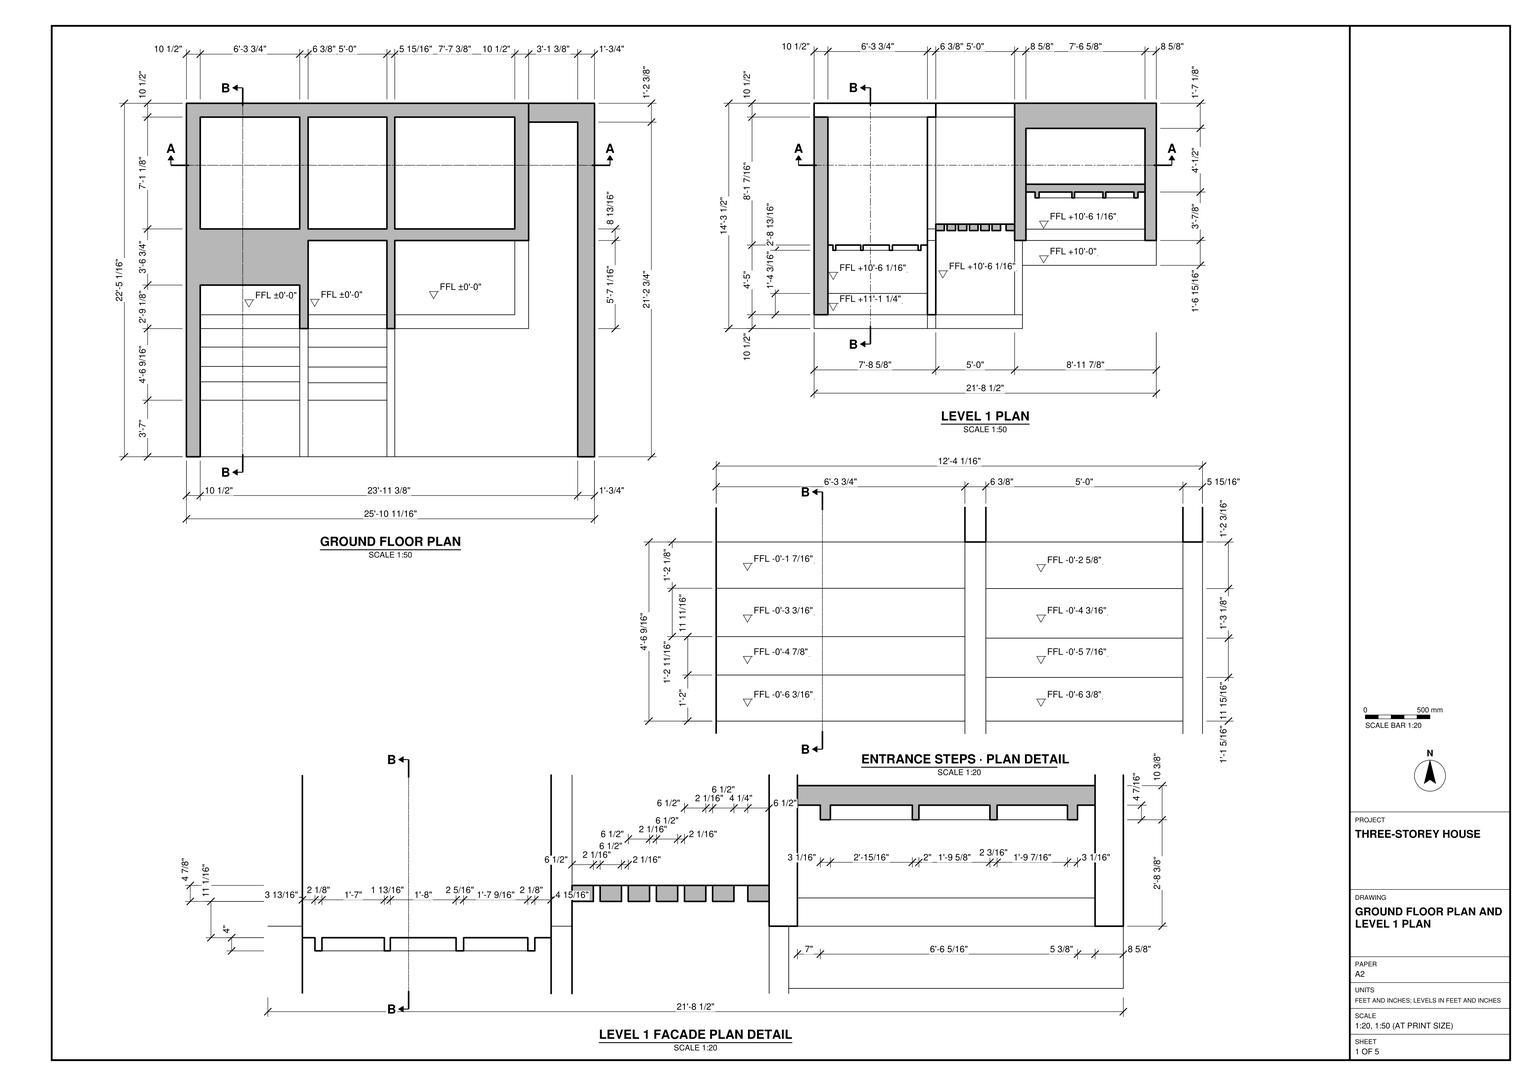
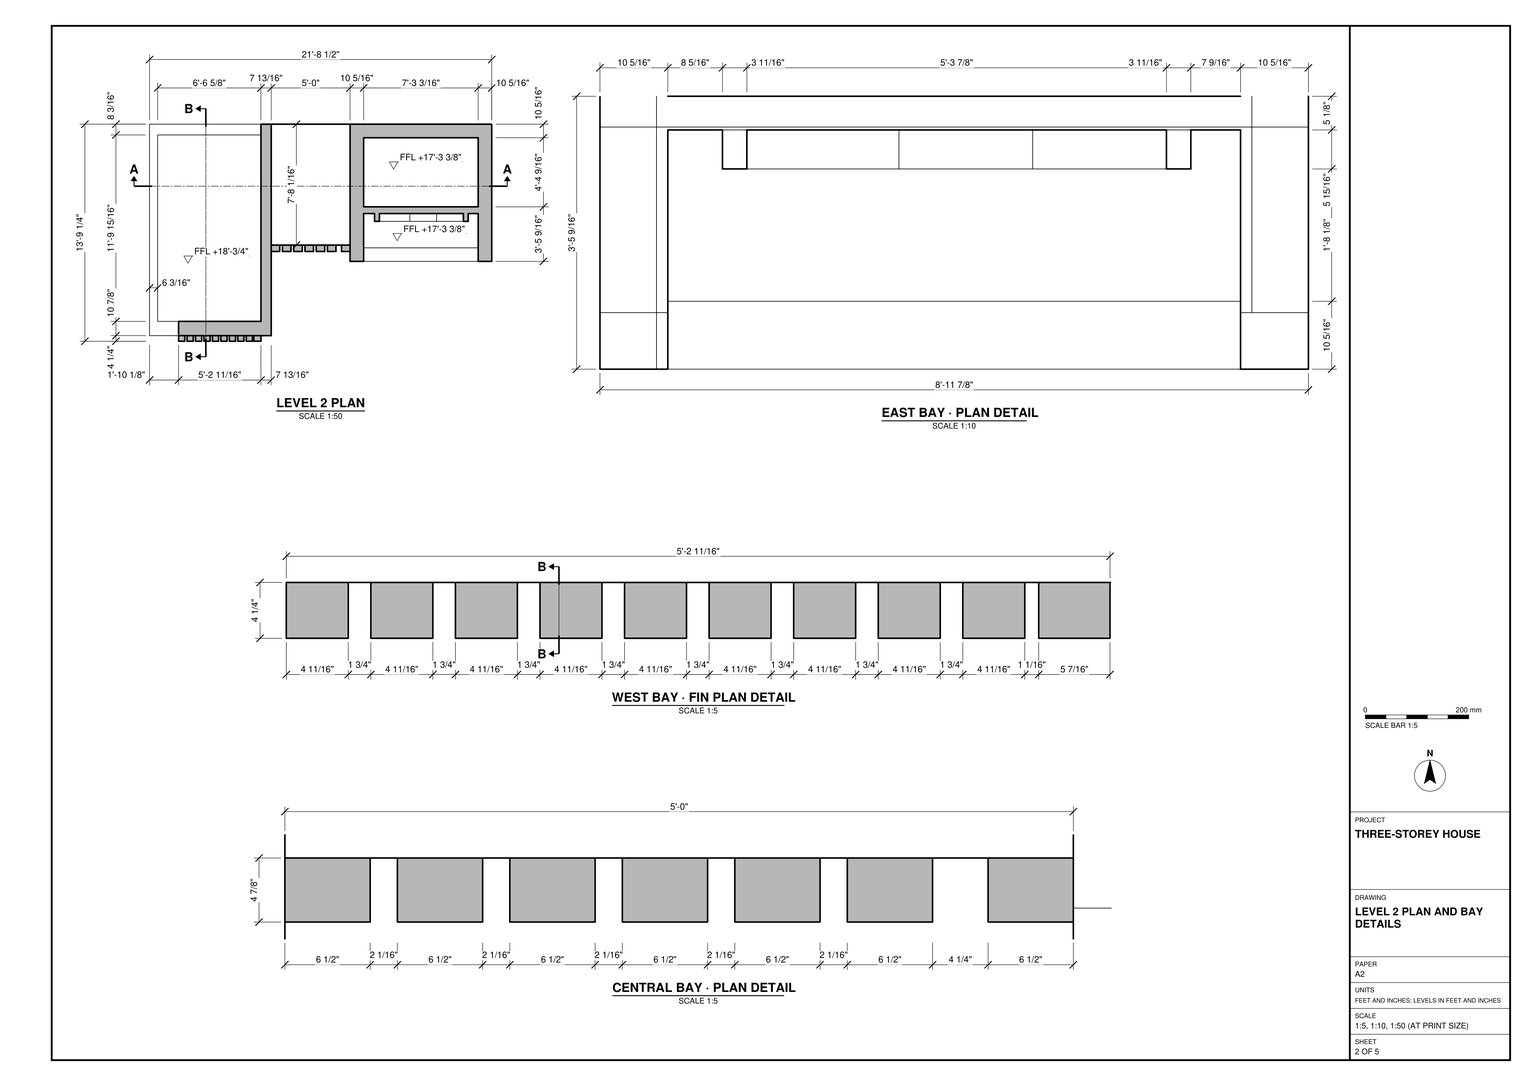
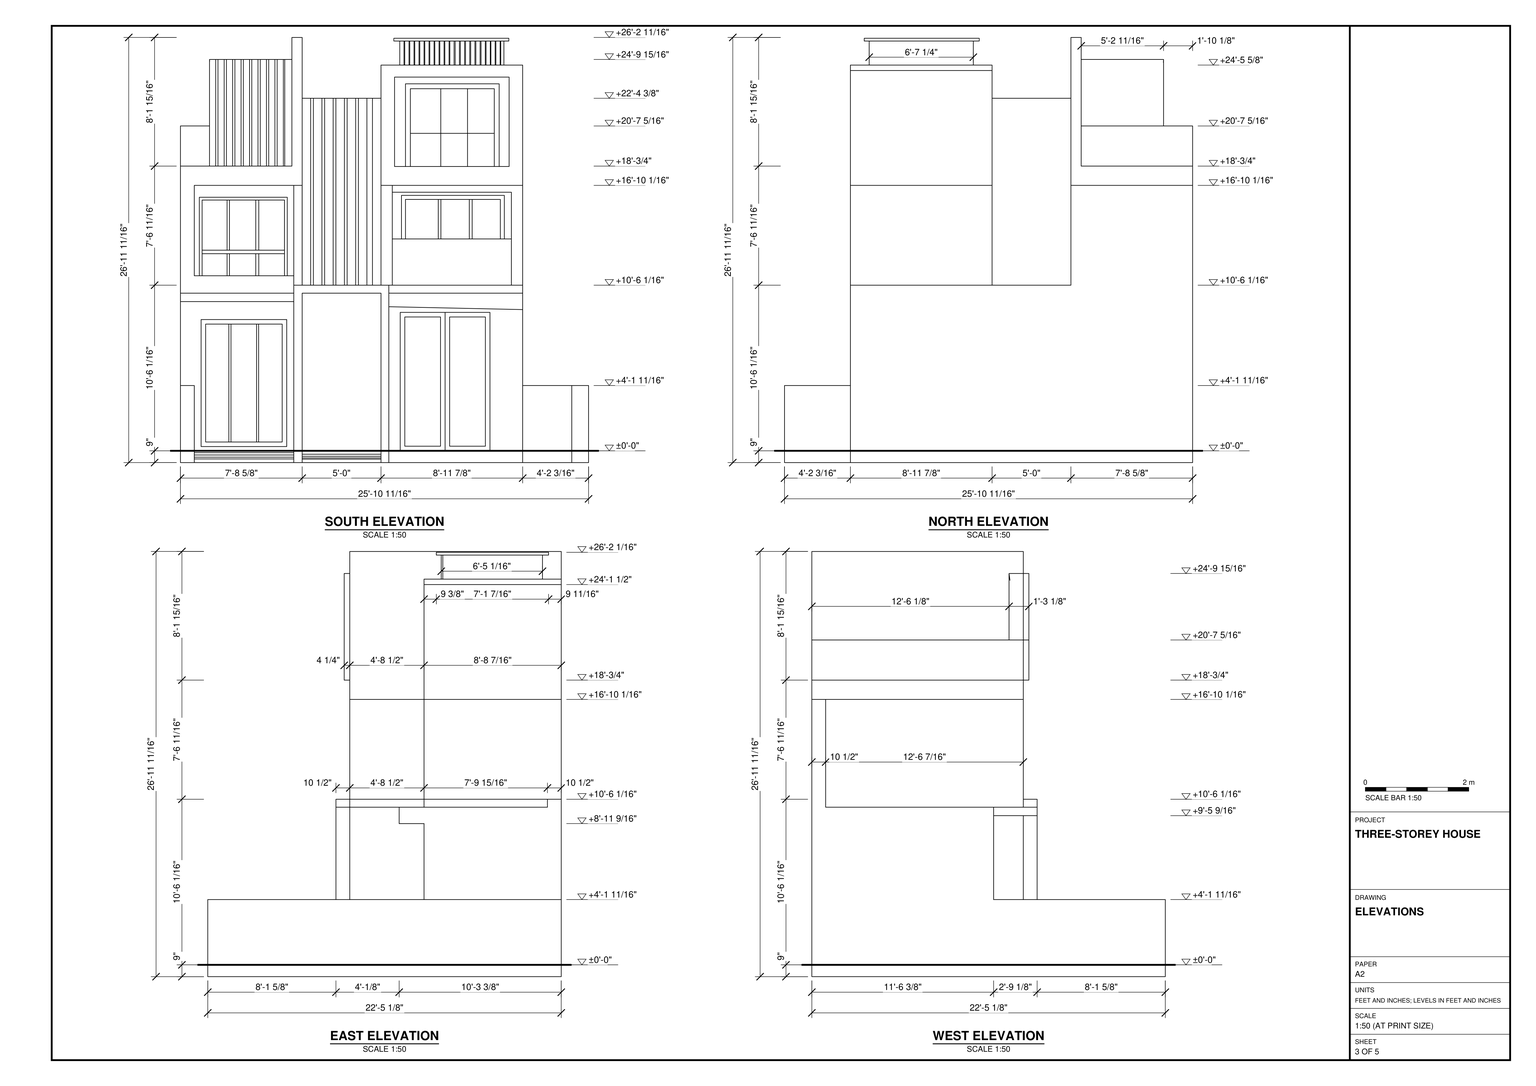
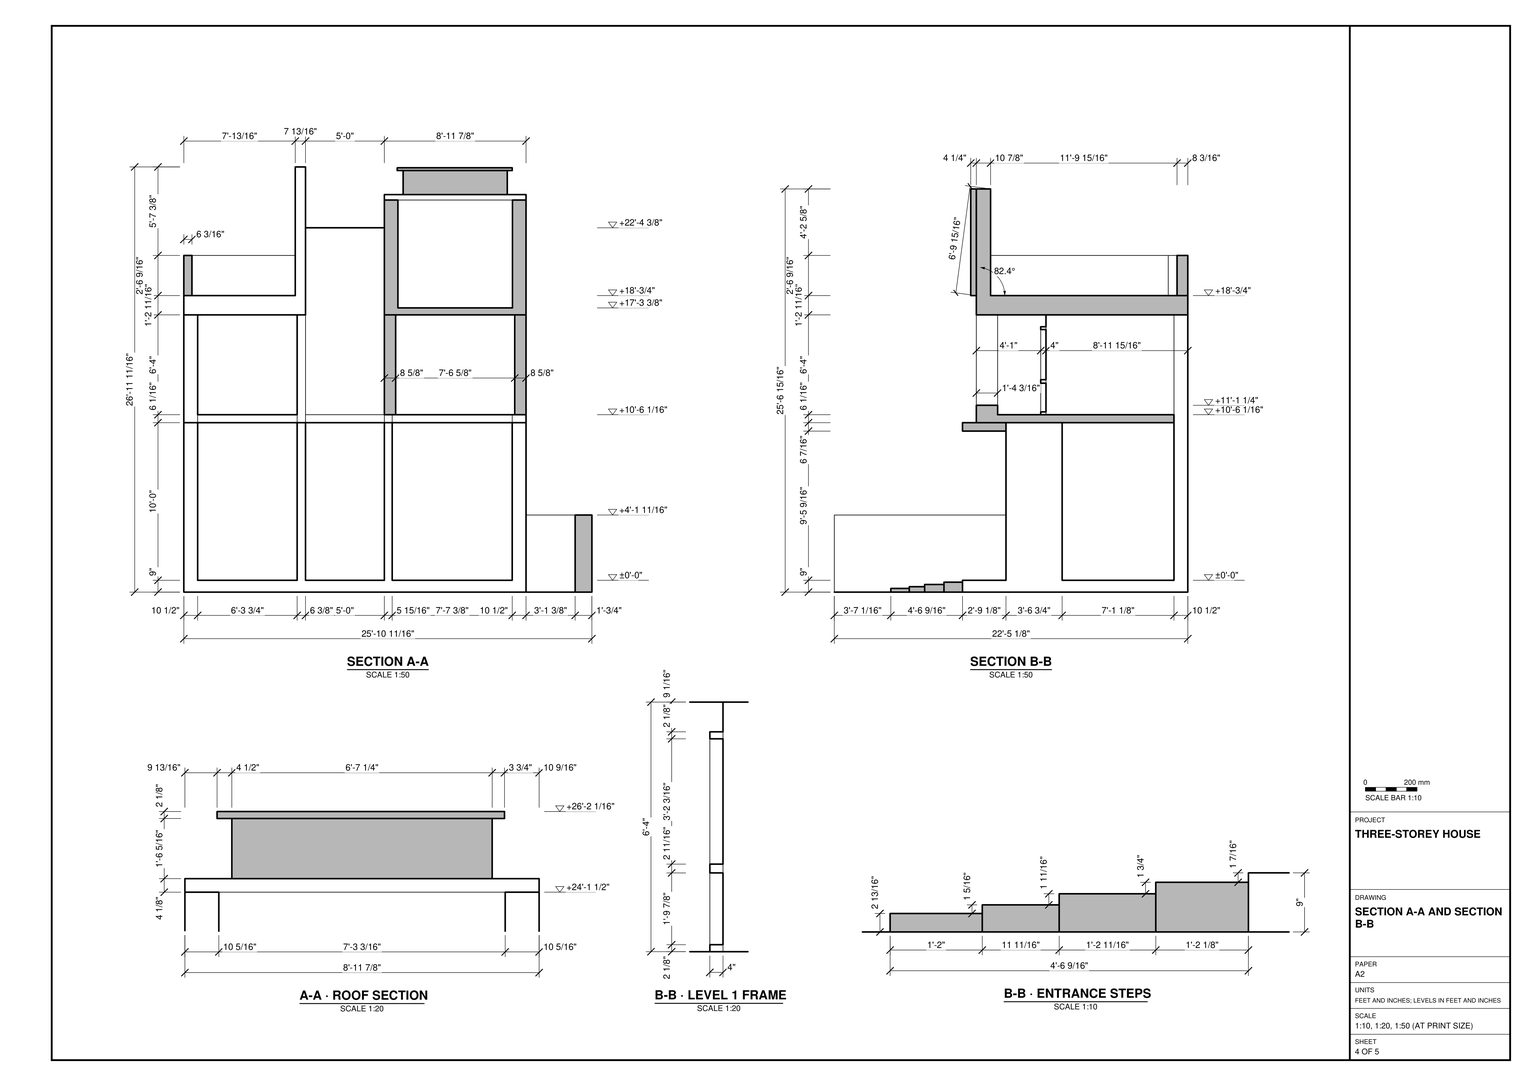
Build the three-storey house shown in task_files/diagram_01.pdf. Work in feet and inches. The overall width is 25'-10 11/16" east to west, the depth is 22'-5 1/16" north to south, and the height from the bottom of the base to the highest point is 26'-11 11/16". Set the ground floor at ±0'-0", Level 1 at +10'-6 1/16", and Level 2 at +18'-3/4".

Start with the ground-floor plan, including the base, the walls flanking the forecourt, and the two adjacent runs of shallow entrance steps. Use the wall thicknesses and partition positions drawn on each plan. Model the floor slabs and follow the stepped outline of the upper floors: the west bay projects furthest south, the centre bay is recessed from it, and the east bay sits further back. Use the south elevation for the arrangement of framed doors and windows, the solid panels below the upper glazing, and the vertical fins. Follow the bay details for the depth and spacing of the fins. Finish the roof with the different wall heights and the raised, capped detail over the east bay.

Keep walls, slabs, stairs, and roof elements in separate groups or components. Keep each furniture or joinery piece shown separate, and use components for repeated parts such as fins. Any decor or loose items shown may be represented by suitable library components. Save one SketchUp model as output_files/three_storey_house_with_stepped_bays_and_facade_fins.skp.

# SketchUp Ruby script. Lengths in inches.
U = 1.inch
M = Sketchup.active_model
def pt(a) = Geom::Point3d.new(a.map { |v| v * U })
def face(e, loops, mat)
  f = e.add_face(loops[0].map { |a| pt(a) })
  loops[1..].each { |l| e.add_face(l.map { |a| pt(a) }).erase! }
  f.material = f.back_material = mat if mat
  f
end
# faces: each face lists its corners as indices into pts; further lists are holes
def faces(e, pts, list, mat = nil) = list.each { |f| face(e, (f[0].is_a?(Array) ? f : [f]).map { |l| l.map { |i| pts[i] } }, mat) }
# xy, xz, yz: faces in a plane at the given z, y or x. An outline is a flat list of corners, or four numbers for a rectangle; further outlines are holes
def ring(l) = l.size == 4 ? [[l[0], l[1]], [l[2], l[1]], [l[2], l[3]], [l[0], l[3]]] : l.each_slice(2).to_a
def flat(e, list, mat, &to3) = list.each { |f| face(e, (f[0].is_a?(Array) ? f : [f]).map { |l| ring(l).map { |u, v| to3.(u, v) } }, mat) }
def xy(e, z, list, mat = nil) = flat(e, list, mat) { |x, y| [x, y, z] }
def xz(e, y, list, mat = nil) = flat(e, list, mat) { |x, z| [x, y, z] }
def yz(e, x, list, mat = nil) = flat(e, list, mat) { |y, z| [x, y, z] }
def lines(e, pts, list) = list.each { |a, b| e.add_line(pt(pts[a]), pt(pts[b])) }
# prism: a flat outline (further loops are holes) pulled along v
def prism(e, loops, v, mat = nil)
  f = face(e, loops, mat); d = Geom::Vector3d.new(v.map { |x| x * U })
  f.pushpull(f.normal.samedirection?(d) ? d.length : -d.length)
end
def box(e, o, s, mat = nil) = prism(e, [[o, [o[0] + s[0], o[1], o[2]], [o[0] + s[0], o[1] + s[1], o[2]], [o[0], o[1] + s[1], o[2]]]], [0, 0, s[2]], mat)
def at(x, y, z, deg = 0) = Geom::Transformation.translation(pt([x, y, z])) * Geom::Transformation.rotation(ORIGIN, Z_AXIS, deg.degrees)
def axes(o, x, y, z) = Geom::Transformation.new([*x, 0, *y, 0, *z, 0, *pt(o).to_a, 1])
def part(name) = M.definitions.add(name)
# library, detail: a bought-in or finely detailed component or shape, given as its bounding box
def library(name, o, s) = part(name).tap { |d| box(d.entities, o, s) }
def detail(e, o, s) = box(e.add_group.entities, o, s)
def put(e, d, t, mat = nil) = e.add_instance(d, t).tap { |i| i.material = mat if mat }
def group(e, t, mat = nil) = e.add_group.tap { |g| g.transformation = t; g.material = mat if mat }.entities
root = M.entities
M.materials.add("[Basic Tile]").color = [203, 206, 202]
M.materials.add("[Blinds Vertical Stripe Gray]").color = [160, 160, 160]
M.materials.add("[Color C01]").color = [255, 229, 204]
M.materials.add("[Formica Graystone]").color = [178, 174, 161]
M.materials.add("[Formica Graystone]1").color = [201, 197, 182]
M.materials.add("[Formica Graystone]3").color = [149, 146, 135]
M.materials.add("[Formica Laminate Dark]").color = [50, 53, 60]
M.materials.add("[Formica Speckled Grey]").color = [94, 105, 111]
M.materials.add("[Terrazzo Tile Light]").color = [219, 217, 210]
M.materials.add("[Translucent Glass Blue]").color = [100, 149, 237]
M.materials["[Translucent Glass Blue]"].alpha = 0.5
M.materials.add("[Translucent Glass Safety]").color = [204, 235, 244]
M.materials["[Translucent Glass Safety]"].alpha = 0.5
M.materials.add("[Translucent Glass Sky Reflection]").color = [126, 138, 183]
M.materials["[Translucent Glass Sky Reflection]"].alpha = 0.52
M.materials.add("[Vegetation Grass Artificial]").color = [98, 140, 74]
M.materials.add("[Wood Cherry Original]").color = [152, 86, 42]
M.materials.add("[Wood Veneer 01]").color = [79, 46, 24]
xy(root,0,[[0,0,0,269.09,260.51,269.09,260.51,97.58,10.52,97.58,10.52,0],[297.89,0,297.89,254.74,260.51,254.74,260.51,269.09,310.66,269.09,310.66,0],[10.52,43.03,86.27,57.06],[92.65,43.03,152.65,56.34],[92.65,56.34,152.65,68.3],
  [10.52,57.06,86.27,68.77],[92.65,68.3,152.65,83.4],[10.52,68.77,86.27,83.48],[92.65,83.4,152.65,97.58],[10.52,83.48,86.27,97.58]])
xy(root,0,[[10.52,0,86.27,43.03],[86.27,0,92.65,97.58],[92.65,0,152.65,43.03],[152.65,0,158.61,97.58],[158.61,0,158.61,97.58,260.51,97.58,260.51,254.74,297.89,254.74,297.89,0]],"[Vegetation Grass Artificial]")
xy(root,2.625,[[92.65,43.03,152.65,56.34]],"[Basic Tile]")
xy(root,2.8125,[[10.52,43.03,86.27,57.06]],"[Basic Tile]")
xy(root,3.5625,[[92.65,56.34,152.65,68.3]],"[Basic Tile]")
xy(root,4.125,[[10.52,57.06,86.27,68.77]],"[Basic Tile]")
xy(root,4.8125,[[92.65,68.3,152.65,83.4]],"[Basic Tile]")
xy(root,5.8125,[[10.52,68.77,86.27,83.48]],"[Basic Tile]")
xy(root,6.375,[[92.65,83.4,152.65,97.58]],"[Basic Tile]")
xy(root,7.5625,[[10.52,83.48,86.27,97.58]],"[Basic Tile]")
xy(root,9,[[10.52,173.43,86.27,258.57],[92.65,173.43,152.65,258.57],[158.61,173.43,249.99,258.57]])
xy(root,9,[[10.52,97.58,86.27,108.11],[92.65,97.58,152.65,108.11],[10.52,108.11,86.27,130.69]],"[Basic Tile]")
xy(root,9,[[92.65,108.11,152.65,164.63]],"[Color C01]")
xy(root,9,[[158.61,97.58,260.51,97.58,260.51,164.63,249.99,164.63,249.99,108.11,158.61,108.11],[158.61,108.11,249.99,164.63]],"[Terrazzo Tile Light]")
xy(root,58.6875,[[0,0,10.52,130.69],[297.89,0,310.66,0,310.66,269.09,260.51,269.09,260.51,254.74,297.89,254.74]],"[Terrazzo Tile Light]")
xy(root,122.58,[[0,97.58,86.27,130.69]])
xy(root,129,[[92.65,97.58,152.65,108.11],[0,108.11,86.27,130.69],[86.27,108.11,92.65,164.63],[92.65,108.11,152.65,164.63],[0,130.69,86.27,164.63],
  [0,164.63,260.51,173.43],[0,173.43,10.52,258.57],[10.52,173.43,86.27,258.57],[86.27,173.43,92.65,258.57],[92.65,173.43,152.65,258.57],
  [152.65,173.43,158.61,258.57],[158.61,173.43,249.99,258.57],[249.99,173.43,260.51,258.57]])
xy(root,129,[[0,97.58,86.27,108.11],[152.65,108.11,158.61,164.63],[158.61,145.69,260.51,164.63]],"[Color C01]")
xy(root,135.0625,[[14.35,157.13,81.31,157.13,81.31,161.13,86.27,161.13,86.27,258.57,10.52,258.57,10.52,161.13,14.35,161.13],[152.65,164.63,152.65,258.57,260.51,258.57,260.51,164.63,251.9,164.63,251.9,249.96,161.26,249.96,161.26,164.63],[161.26,164.63,251.9,173.24],[92.63,172.17,99.12,177.05],[101.19,172.17,107.68,177.05],
  [109.75,172.17,116.25,177.05],[118.32,172.17,124.81,177.05],[126.88,172.17,133.37,177.05],[135.44,172.17,141.93,177.05],[146.16,172.17,152.65,177.05],
  [161.26,173.24,251.9,201.49],[161.26,207.44,251.9,249.96],[92.65,258.57,152.65,269.09],[152.65,258.57,158.61,269.09],[158.61,258.57,249.99,269.09],
  [249.99,258.57,260.51,269.09]])
xy(root,135.0625,[[86.27,97.58,92.62,108.11],[92.62,97.58,158.61,108.11],[92.62,108.11,152.65,108.11,152.65,172.17,146.16,172.17,146.16,177.05,141.93,177.05,141.93,172.17,135.44,172.17,135.44,177.05,133.37,177.05,133.37,172.17,126.88,172.17,126.88,177.05,124.81,177.05,124.81,172.17,118.32,172.17,118.32,177.05,116.25,177.05,116.25,172.17,109.75,172.17,109.75,177.05,107.68,177.05,107.68,172.17,101.19,172.17,101.19,177.05,99.12,177.05,99.12,172.17,92.63,172.17],[10.52,124.32,86.27,124.32,86.27,161.13,81.31,161.13,81.31,157.13,14.35,157.13,14.35,161.13,10.52,161.13]],"[Color C01]")
xy(root,137.12,[[168.24,197.05,246.55,201.49]])
xy(root,137.19,[[16.48,157.13,35.48,161.13],[37.3,157.13,57.33,161.13],[59.62,157.13,79.18,161.13]],"[Wood Veneer 01]")
xy(root,140.17,[[171.3,197.05,196.26,201.49],[198.27,197.05,219.88,201.49],[222.0625,197.05,243.5,201.49]],"[Wood Veneer 01]")
xy(root,142.25,[[10.52,108.11,86.27,124.32]],"[Color C01]")
xy(root,159.05,[[16.48,157.13,35.48,161.13],[37.3,157.13,57.33,161.13],[59.62,157.13,79.18,161.13]])
xy(root,161.73,[[16.48,157.13,35.48,161.13],[37.3,157.13,57.33,161.13],[59.62,157.13,79.18,161.13]],"[Wood Veneer 01]")
xy(root,170.28,[[161.26,164.63,251.9,173.24]],"[Translucent Glass Safety]")
xy(root,199.89,[[16.48,157.13,35.48,161.13],[37.3,157.13,57.33,161.13],[59.62,157.13,79.18,161.13]],"[Wood Veneer 01]")
xy(root,200.375,[[171.3,197.05,196.26,201.49],[198.27,197.05,219.88,201.49],[222.0625,197.05,243.5,201.49]])
xy(root,202.01,[[14.35,157.13,81.31,161.13]],"[Wood Veneer 01]")
xy(root,203.43,[[168.24,197.05,246.55,201.49]],"[Wood Veneer 01]")
xy(root,205.84,[[161.26,164.63,251.9,173.24]],"[Wood Cherry Original]")
xy(root,211.0625,[[86.27,108.11,92.62,124.32],[92.62,108.11,92.63,124.32],[0,124.32,10.52,258.57],[86.27,124.32,92.62,124.32,92.63,172.17,92.63,258.57,86.27,258.57],[92.62,124.32,92.63,172.17,92.63,124.32],
  [10.52,161.13,86.27,161.13,86.27,258.57,92.63,258.57,92.63,269.09,0,269.09,0,258.57,10.52,258.57],[152.65,164.63,161.26,173.24],[161.26,164.63,260.51,173.24],[152.65,173.24,161.26,201.49],[251.9,173.24,260.51,201.49],
  [92.63,177.05,92.65,258.57,92.63,258.57],[152.65,201.49,161.26,207.44],[161.26,201.49,251.9,207.44],[251.9,201.49,260.51,207.44],[152.65,207.44,161.26,269.09],
  [161.26,207.44,251.9,249.96],[251.9,207.44,260.51,269.09],[161.26,249.96,251.9,269.09],[92.63,258.57,92.65,269.09]])
xy(root,211.0625,[[10.52,108.11,86.27,161.13]],"[Color C01]")
xy(root,216.375,[[162.98,174.96,250.18,201.05]],"[Color C01]")
xy(root,216.375,[[162.98,206.18,250.18,258.76]],"[Formica Graystone]1")
xy(root,219.3125,[[171.3,195.11,242.61,201.05]])
xy(root,223.03,[[175.02,195.11,198.17,201.05],[198.17,195.11,218.53,201.05],[218.53,195.11,238.9,201.05]],"[Wood Veneer 01]")
xy(root,225.4375,[[162.98,164.63,250.18,174.96]],"[Color C01]")
xy(root,225.75,[[22.12,103.86,26.83,108.11],[28.55,103.86,33.27,108.11],[34.99,103.86,39.71,108.11],[41.43,103.86,46.15,108.11],[47.87,103.86,52.58,108.11],
  [54.3,103.86,59.02,108.11],[60.74,103.86,65.46,108.11],[67.18,103.86,71.9,108.11],[73.62,103.86,78.33,108.11],[79.39,103.86,84.82,108.11],
  [0,108.11,0,269.09,84.82,269.09,84.82,260.9,6.18,260.9,6.18,118.96,22.12,118.96,22.12,108.11],[6.18,118.96,84.82,260.9]])
xy(root,256.3125,[[0,108.11,22.12,108.11,22.12,118.96,6.18,118.96,6.18,260.9,84.82,260.9,84.82,269.09,0,269.09]],"[Color C01]")
xy(root,277.375,[[92.63,172.17,99.12,177.05],[101.19,172.17,107.68,177.05],[109.75,172.17,116.25,177.05],[118.32,172.17,124.81,177.05],[126.88,172.17,133.37,177.05],
  [135.44,172.17,141.93,177.05],[146.16,172.17,152.65,177.05]])
xy(root,277.375,[[92.63,177.05,152.65,177.05,152.65,269.09,92.65,269.09]],"[Formica Speckled Grey]")
xy(root,284.66,[[175.02,195.11,198.17,201.05],[198.17,195.11,218.53,201.05],[218.53,195.11,238.9,201.05]],"[Wood Veneer 01]")
xy(root,288.375,[[171.3,195.11,242.61,201.05]],"[Wood Veneer 01]")
xy(root,293.5,[[162.98,164.63,250.18,201.05]],"[Color C01]")
xy(root,298.5,[[152.65,201.05,260.51,206.18],[152.65,206.18,162.98,269.09],[250.18,206.18,260.51,269.09],[162.98,258.76,250.18,269.09]])
xy(root,302.625,[[166.94,177.73,170.16,178.92],[170.76,177.73,173.97,178.92],[174.57,177.73,177.78,178.92],[178.38,177.73,181.6,178.92],[182.19,177.73,185.41,178.92],
  [186.01,177.73,189.22,178.92],[189.82,177.73,193.03,178.92],[193.63,177.73,196.85,178.92],[197.44,177.73,200.66,178.92],[201.26,177.73,204.47,178.92],
  [205.07,177.73,208.28,178.92],[209.13,177.73,212.35,178.92],[213.07,177.73,216.28,178.92],[217.01,177.73,220.22,178.92],[220.94,177.73,224.16,178.92],
  [224.88,177.73,228.1,178.92],[228.82,177.73,232.03,178.92],[232.63,177.73,235.85,178.92],[236.32,177.73,239.53,178.92],[240.13,177.73,243.35,178.92],
  [243.83,177.73,246.22,178.92],[166.94,178.92,246.22,254.8]])
xy(root,302.625,[[[152.65,164.63,260.51,269.09],[166.94,177.73,166.94,254.8,246.22,254.8,246.22,177.73,243.83,177.73,243.83,178.92,243.35,178.92,243.35,177.73,240.13,177.73,240.13,178.92,239.53,178.92,239.53,177.73,236.32,177.73,236.32,178.92,235.85,178.92,235.85,177.73,232.63,177.73,232.63,178.92,232.03,178.92,232.03,177.73,228.82,177.73,228.82,178.92,228.1,178.92,228.1,177.73,224.88,177.73,224.88,178.92,224.16,178.92,224.16,177.73,220.94,177.73,220.94,178.92,220.22,178.92,220.22,177.73,217.01,177.73,217.01,178.92,216.28,178.92,216.28,177.73,213.07,177.73,213.07,178.92,212.35,178.92,212.35,177.73,209.13,177.73,209.13,178.92,208.28,178.92,208.28,177.73,205.07,177.73,205.07,178.92,204.47,178.92,204.47,177.73,201.26,177.73,201.26,178.92,200.66,178.92,200.66,177.73,197.44,177.73,197.44,178.92,196.85,178.92,196.85,177.73,193.63,177.73,193.63,178.92,193.03,178.92,193.03,177.73,189.82,177.73,189.82,178.92,189.22,178.92,189.22,177.73,186.01,177.73,186.01,178.92,185.41,178.92,185.41,177.73,182.19,177.73,182.19,178.92,181.6,178.92,181.6,177.73,178.38,177.73,178.38,178.92,177.78,178.92,177.78,177.73,174.57,177.73,174.57,178.92,173.97,178.92,173.97,177.73,170.76,177.73,170.76,178.92,170.16,178.92,170.16,177.73]]],"[Color C01]")
xy(root,306.9375,[[22.12,103.86,26.83,108.11],[28.55,103.86,33.27,108.11],[34.99,103.86,39.71,108.11],[41.43,103.86,46.15,108.11],[47.87,103.86,52.58,108.11],
  [54.3,103.86,59.02,108.11],[60.74,103.86,65.46,108.11],[67.18,103.86,71.9,108.11],[73.62,103.86,78.33,108.11],[79.39,103.86,84.82,108.11],
  [22.12,108.11,84.82,118.96]],"[Formica Graystone]")
xy(root,320.9375,[[162.44,173.98,162.44,259.42,246.22,259.42,246.22,254.8,166.94,254.8,166.94,177.73,170.16,177.73,170.16,178.92,170.76,178.92,170.76,177.73,173.97,177.73,173.97,178.92,174.57,178.92,174.57,177.73,177.78,177.73,177.78,178.92,178.38,178.92,178.38,177.73,181.6,177.73,181.6,178.92,182.19,178.92,182.19,177.73,185.41,177.73,185.41,178.92,186.01,178.92,186.01,177.73,189.22,177.73,189.22,178.92,189.82,178.92,189.82,177.73,193.03,177.73,193.03,178.92,193.63,178.92,193.63,177.73,196.85,177.73,196.85,178.92,197.44,178.92,197.44,177.73,200.66,177.73,200.66,178.92,201.26,178.92,201.26,177.73,204.47,177.73,204.47,178.92,205.07,178.92,205.07,177.73,208.28,177.73,208.28,178.92,209.13,178.92,209.13,177.73,212.35,177.73,212.35,178.92,213.07,178.92,213.07,177.73,216.28,177.73,216.28,178.92,217.01,178.92,217.01,177.73,220.22,177.73,220.22,178.92,220.94,178.92,220.94,177.73,224.16,177.73,224.16,178.92,224.88,178.92,224.88,177.73,228.1,177.73,228.1,178.92,228.82,178.92,228.82,177.73,232.03,177.73,232.03,178.92,232.63,178.92,232.63,177.73,235.85,177.73,235.85,178.92,236.32,178.92,236.32,177.73,239.53,177.73,239.53,178.92,240.13,178.92,240.13,177.73,243.35,177.73,243.35,178.92,243.83,178.92,243.83,177.73,246.22,177.73,246.22,259.42,249.97,259.42,249.97,173.98],[166.94,177.73,170.16,178.92],[170.76,177.73,173.97,178.92],[174.57,177.73,177.78,178.92],[178.38,177.73,181.6,178.92],
  [182.19,177.73,185.41,178.92],[186.01,177.73,189.22,178.92],[189.82,177.73,193.03,178.92],[193.63,177.73,196.85,178.92],[197.44,177.73,200.66,178.92],
  [201.26,177.73,204.47,178.92],[205.07,177.73,208.28,178.92],[209.13,177.73,212.35,178.92],[213.07,177.73,216.28,178.92],[217.01,177.73,220.22,178.92],
  [220.94,177.73,224.16,178.92],[224.88,177.73,228.1,178.92],[228.82,177.73,232.03,178.92],[232.63,177.73,235.85,178.92],[236.32,177.73,239.53,178.92],
  [240.13,177.73,243.35,178.92],[243.83,177.73,246.22,178.92],[166.94,178.92,246.22,254.8]])
xy(root,323.0625,[[162.44,173.98,249.97,259.42]],"[Formica Speckled Grey]")
xy(root,323.6875,[[84.82,108.11,92.63,269.09]],"[Color C01]")
xz(root,0,[[0,0,10.52,58.6875],[297.89,0,310.66,58.6875]],"[Terrazzo Tile Light]")
xz(root,43.03,[[10.52,0,86.27,2.8125],[92.65,0,152.65,2.625]],"[Basic Tile]")
xz(root,56.34,[[92.65,0,152.65,2.625]])
xz(root,56.34,[[92.65,2.625,152.65,3.5625]],"[Basic Tile]")
xz(root,57.06,[[10.52,0,86.27,2.8125]])
xz(root,57.06,[[10.52,2.8125,86.27,4.125]],"[Basic Tile]")
xz(root,68.3,[[92.65,0,152.65,3.5625]])
xz(root,68.3,[[92.65,3.5625,152.65,4.8125]],"[Basic Tile]")
xz(root,68.77,[[10.52,0,86.27,4.125]])
xz(root,68.77,[[10.52,4.125,86.27,5.8125]],"[Basic Tile]")
xz(root,83.4,[[92.65,0,152.65,4.8125]])
xz(root,83.4,[[92.65,4.8125,152.65,6.375]],"[Basic Tile]")
xz(root,83.48,[[10.52,0,86.27,5.8125]])
xz(root,83.48,[[10.52,5.8125,86.27,7.5625]],"[Basic Tile]")
xz(root,97.58,[[10.52,0,86.27,7.5625],[92.65,0,152.65,6.375]])
xz(root,97.58,[[92.65,6.375,152.65,9],[10.52,7.5625,86.27,9]],"[Basic Tile]")
xz(root,97.58,[[86.27,0,92.65,0,92.65,129,152.65,129,152.65,0,158.61,0,158.61,135.0625,86.27,135.0625],[0,122.58,86.27,129]],"[Color C01]")
xz(root,97.58,[[158.61,0,260.51,9]],"[Terrazzo Tile Light]")
xz(root,103.86,[[22.12,225.75,26.83,306.9375],[28.55,225.75,33.27,306.9375],[34.99,225.75,39.71,306.9375],[41.43,225.75,46.15,306.9375],[47.87,225.75,52.58,306.9375],
  [54.3,225.75,59.02,306.9375],[60.74,225.75,65.46,306.9375],[67.18,225.75,71.9,306.9375],[73.62,225.75,78.33,306.9375],[79.39,225.75,84.82,306.9375]],"[Formica Graystone]")
xz(root,108.11,[[86.27,129,152.65,135.0625],[152.65,129,158.61,135.0625],[22.12,225.75,26.83,306.9375],[28.55,225.75,33.27,306.9375],[34.99,225.75,39.71,306.9375],
  [41.43,225.75,46.15,306.9375],[47.87,225.75,52.58,306.9375],[54.3,225.75,59.02,306.9375],[60.74,225.75,65.46,306.9375],[67.18,225.75,71.9,306.9375],
  [73.62,225.75,78.33,306.9375],[79.39,225.75,84.82,306.9375]])
xz(root,108.11,[[0,129,86.27,129,86.27,142.25,10.52,142.25,10.52,211.0625,92.63,211.0625,92.63,323.6875,84.82,323.6875,84.82,225.75,0,225.75],[86.27,135.0625,92.62,211.0625],[0,225.75,22.12,256.3125]],"[Color C01]")
xz(root,108.11,[[26.83,225.75,28.55,306.9375],[33.27,225.75,34.99,306.9375],[39.71,225.75,41.43,306.9375],[46.15,225.75,47.87,306.9375],[52.58,225.75,54.3,306.9375],
  [59.02,225.75,60.74,306.9375],[65.46,225.75,67.18,306.9375],[71.9,225.75,73.62,306.9375],[78.33,225.75,79.39,306.9375]],"[Formica Laminate Dark]")
xz(root,118.96,[[6.18,225.75,22.12,256.3125],[22.12,225.75,84.82,306.9375]],"[Formica Graystone]3")
xz(root,124.32,[[10.52,135.0625,86.27,142.25]])
xz(root,130.69,[[0,122.58,86.27,129]])
xz(root,130.69,[[19.18,15.7,36.83,105.45],[38.46,15.7,57.95,105.45],[59.51,15.7,77.43,105.45]],"[Blinds Vertical Stripe Gray]")
xz(root,130.69,[[[10.52,9,86.27,9,86.27,122.58,0,122.58,0,58.6875,10.52,58.6875],[15.71,12.23,80.9,108.92]]],"[Color C01]")
xz(root,130.69,[[[15.71,12.23,80.9,108.92],[19.18,15.7,77.43,105.45]],[36.83,15.7,38.46,105.45],[57.95,15.7,59.51,105.45]],"[Wood Veneer 01]")
xz(root,145.69,[[260.51,116.51,260.51,129,158.61,129,158.61,118.6875]],"[Color C01]")
xz(root,157.13,[[[14.35,135.0625,81.31,202.01],[16.48,137.19,79.18,199.89]],[35.48,137.19,37.3,159.05],[57.33,137.19,59.62,159.05],[16.48,159.05,79.18,161.73],[35.48,161.73,37.3,199.89],
  [57.33,161.73,59.62,199.89]],"[Wood Veneer 01]")
xz(root,161.13,[[10.52,135.0625,14.35,135.0625,14.35,202.01,81.31,202.01,81.31,135.0625,86.27,135.0625,86.27,211.0625,10.52,211.0625]],"[Color C01]")
xz(root,161.13,[[16.48,137.19,35.48,159.05],[37.3,137.19,57.33,159.05],[59.62,137.19,79.18,159.05],[16.48,161.73,35.48,199.89],[37.3,161.73,57.33,199.89],
  [59.62,161.73,79.18,199.89]],"[Translucent Glass Blue]")
xz(root,164.63,[[170.77,12.48,197.96,110.89],[204.93,12.48,232.12,110.89]],"[Blinds Vertical Stripe Gray]")
xz(root,164.63,[[158.61,9,167.29,9,167.29,114.375,235.6,114.375,235.6,9,260.51,9,260.51,116.51,158.61,118.6875],[152.65,135.0625,161.26,211.0625],[[152.65,211.0625,260.51,302.625],[162.98,225.4375,250.18,293.5]]],"[Color C01]")
xz(root,164.63,[[152.65,129,260.51,135.0625]],"[Formica Speckled Grey]")
xz(root,164.63,[[92.65,9,152.65,129],[161.26,135.0625,251.9,170.28]],"[Translucent Glass Safety]")
xz(root,164.63,[[251.9,135.0625,260.51,135.0625,260.51,211.0625,161.26,211.0625,161.26,205.84,251.9,205.84]],"[Wood Cherry Original]")
xz(root,164.63,[[[167.29,9,201.45,114.375],[170.77,12.48,197.96,110.89]],[[201.45,9,235.6,114.375],[204.93,12.48,232.12,110.89]]],"[Wood Veneer 01]")
xz(root,172.17,[[92.63,135.0625,99.12,277.375],[101.19,135.0625,107.68,277.375],[109.75,135.0625,116.25,277.375],[118.32,135.0625,124.81,277.375],[126.88,135.0625,133.37,277.375],
  [135.44,135.0625,141.93,277.375],[146.16,135.0625,152.65,277.375]],"[Formica Graystone]")
xz(root,173.24,[[161.26,135.0625,251.9,170.28]],"[Translucent Glass Safety]")
xz(root,173.24,[[161.26,205.84,251.9,211.0625]],"[Wood Cherry Original]")
xz(root,173.43,[[10.52,9,86.27,129],[92.65,9,152.65,129],[158.61,9,249.99,129]])
xz(root,173.98,[[162.44,320.9375,249.97,323.0625]],"[Formica Speckled Grey]")
xz(root,174.96,[[162.98,216.375,250.18,225.4375]],"[Formica Graystone]1")
xz(root,177.05,[[92.63,135.0625,99.12,277.375],[101.19,135.0625,107.68,277.375],[109.75,135.0625,116.25,277.375],[118.32,135.0625,124.81,277.375],[126.88,135.0625,133.37,277.375],
  [135.44,135.0625,141.93,277.375],[146.16,135.0625,152.65,277.375]])
xz(root,177.05,[[99.12,135.0625,101.19,277.375],[107.68,135.0625,109.75,277.375],[116.25,135.0625,118.32,277.375],[124.81,135.0625,126.88,277.375],[133.37,135.0625,135.44,277.375],
  [141.93,135.0625,146.16,277.375]],"[Formica Laminate Dark]")
xz(root,177.73,[[166.94,302.625,170.16,320.9375],[170.76,302.625,173.97,320.9375],[174.57,302.625,177.78,320.9375],[178.38,302.625,181.6,320.9375],[182.19,302.625,185.41,320.9375],
  [186.01,302.625,189.22,320.9375],[189.82,302.625,193.03,320.9375],[193.63,302.625,196.85,320.9375],[197.44,302.625,200.66,320.9375],[201.26,302.625,204.47,320.9375],
  [205.07,302.625,208.28,320.9375],[209.13,302.625,212.35,320.9375],[213.07,302.625,216.28,320.9375],[217.01,302.625,220.22,320.9375],[220.94,302.625,224.16,320.9375],
  [224.88,302.625,228.1,320.9375],[228.82,302.625,232.03,320.9375],[232.63,302.625,235.85,320.9375],[236.32,302.625,239.53,320.9375],[240.13,302.625,243.35,320.9375],
  [243.83,302.625,246.22,320.9375]],"[Formica Graystone]3")
xz(root,178.92,[[166.94,302.625,170.16,320.9375],[170.16,302.625,170.76,320.9375],[170.76,302.625,173.97,320.9375],[173.97,302.625,174.57,320.9375],[174.57,302.625,177.78,320.9375],
  [177.78,302.625,178.38,320.9375],[178.38,302.625,181.6,320.9375],[181.6,302.625,182.19,320.9375],[182.19,302.625,185.41,320.9375],[185.41,302.625,186.01,320.9375],
  [186.01,302.625,189.22,320.9375],[189.22,302.625,189.82,320.9375],[189.82,302.625,193.03,320.9375],[193.03,302.625,193.63,320.9375],[193.63,302.625,196.85,320.9375],
  [196.85,302.625,197.44,320.9375],[197.44,302.625,200.66,320.9375],[200.66,302.625,201.26,320.9375],[201.26,302.625,204.47,320.9375],[204.47,302.625,205.07,320.9375],
  [205.07,302.625,208.28,320.9375],[208.28,302.625,209.13,320.9375],[209.13,302.625,212.35,320.9375],[212.35,302.625,213.07,320.9375],[213.07,302.625,216.28,320.9375],
  [216.28,302.625,217.01,320.9375],[217.01,302.625,220.22,320.9375],[220.22,302.625,220.94,320.9375],[220.94,302.625,224.16,320.9375],[224.16,302.625,224.88,320.9375],
  [224.88,302.625,228.1,320.9375],[228.1,302.625,228.82,320.9375],[228.82,302.625,232.03,320.9375],[232.03,302.625,232.63,320.9375],[232.63,302.625,235.85,320.9375],
  [235.85,302.625,236.32,320.9375],[236.32,302.625,239.53,320.9375],[239.53,302.625,240.13,320.9375],[240.13,302.625,243.35,320.9375],[243.35,302.625,243.83,320.9375],
  [243.83,302.625,246.22,320.9375]])
xz(root,195.11,[[[171.3,219.3125,242.61,288.375],[175.02,223.03,238.9,284.66]]],"[Wood Veneer 01]")
xz(root,197.05,[[[168.24,137.12,246.55,203.43],[171.3,140.17,243.5,200.375]],[196.26,140.17,198.27,200.375],[219.88,140.17,222.0625,200.375]],"[Wood Veneer 01]")
xz(root,201.05,[[162.98,293.5,250.18,298.5]])
xz(root,201.05,[[[162.98,216.375,250.18,293.5],[171.3,219.3125,242.61,288.375]]],"[Formica Speckled Grey]")
xz(root,201.05,[[175.02,223.03,198.17,250.66],[198.17,223.03,218.53,250.66],[218.53,223.03,238.9,250.66],[175.02,250.66,198.17,284.66],[198.17,250.66,218.53,284.66],
  [218.53,250.66,238.9,284.66]],"[Translucent Glass Sky Reflection]")
xz(root,201.49,[[[161.26,135.0625,251.9,211.0625],[168.24,137.12,246.55,203.43]]],"[Color C01]")
xz(root,201.49,[[171.3,140.17,196.26,200.375],[198.27,140.17,219.88,200.375],[222.0625,140.17,243.5,200.375]],"[Translucent Glass Safety]")
xz(root,206.18,[[162.98,216.375,250.18,298.5]],"[Formica Graystone]1")
xz(root,207.44,[[161.26,135.0625,251.9,211.0625]])
xz(root,249.96,[[161.26,135.0625,251.9,211.0625]])
xz(root,254.74,[[260.51,0,297.89,58.6875]],"[Terrazzo Tile Light]")
xz(root,254.8,[[166.94,302.625,246.22,320.9375]],"[Formica Speckled Grey]")
xz(root,258.57,[[10.52,9,86.27,129],[92.65,9,152.65,129],[158.61,9,249.99,129],[0,129,10.52,211.0625],[10.52,129,86.27,135.0625],
  [86.27,129,92.65,211.0625],[92.65,129,152.65,135.0625],[152.65,129,158.61,135.0625],[158.61,129,249.99,135.0625],[249.99,129,260.51,135.0625]])
xz(root,258.76,[[162.98,216.375,250.18,298.5]])
xz(root,259.42,[[162.44,320.9375,249.97,323.0625]],"[Formica Speckled Grey]")
xz(root,260.9,[[6.18,225.75,84.82,256.3125]],"[Color C01]")
xz(root,269.09,[[0,0,0,211.0625,92.65,211.0625,92.65,135.0625,260.51,135.0625,260.51,0],[92.65,135.0625,152.65,277.375],[152.65,135.0625,260.51,211.0625],[0,211.0625,0,225.75,84.82,225.75,84.82,323.6875,92.63,323.6875,92.63,211.0625],[152.65,211.0625,260.51,298.5],
  [0,225.75,84.82,256.3125],[152.65,298.5,260.51,302.625]],"[Color C01]")
xz(root,269.09,[[260.51,0,310.66,58.6875]],"[Terrazzo Tile Light]")
yz(root,0,[[97.58,122.58,130.69,129],[108.11,129,258.57,211.0625],[108.11,211.0625,269.09,225.75],[108.11,225.75,269.09,256.3125]],"[Color C01]")
yz(root,0,[[0,0,0,58.6875,130.69,58.6875,130.69,129,258.57,129,258.57,211.0625,269.09,211.0625,269.09,0]],"[Terrazzo Tile Light]")
yz(root,6.18,[[118.96,225.75,254.21,256.3125],[254.21,225.75,260.9,256.3125]],"[Color C01]")
yz(root,10.52,[[43.03,0,57.06,2.8125],[57.06,0,68.77,4.125],[68.77,0,83.48,5.8125],[83.48,0,97.58,7.5625],[173.43,9,258.57,129],
  [161.13,135.0625,258.57,211.0625]])
yz(root,10.52,[[124.32,135.0625,161.13,211.0625],[108.11,142.25,124.32,211.0625]],"[Color C01]")
yz(root,10.52,[[0,0,43.03,0,43.03,2.8125,57.06,2.8125,57.06,4.125,68.77,4.125,68.77,5.8125,83.48,5.8125,83.48,7.5625,97.58,7.5625,97.58,9,130.69,9,130.69,58.6875,0,58.6875]],"[Terrazzo Tile Light]")
yz(root,14.35,[[157.13,135.0625,161.13,202.01]],"[Wood Veneer 01]")
yz(root,16.48,[[157.13,137.19,161.13,159.05],[157.13,161.73,161.13,199.89]],"[Wood Veneer 01]")
yz(root,22.12,[[108.11,225.75,118.96,256.3125]])
yz(root,22.12,[[103.86,225.75,108.11,256.3125],[103.86,256.3125,108.11,306.9375],[108.11,256.3125,118.96,306.9375]],"[Formica Graystone]")
yz(root,26.83,[[103.86,225.75,108.11,306.9375]],"[Formica Graystone]1")
yz(root,28.55,[[103.86,225.75,108.11,306.9375]],"[Formica Graystone]")
yz(root,33.27,[[103.86,225.75,108.11,306.9375]],"[Formica Graystone]1")
yz(root,34.99,[[103.86,225.75,108.11,306.9375]],"[Formica Graystone]")
yz(root,35.48,[[157.13,137.19,161.13,159.05],[157.13,161.73,161.13,199.89]],"[Wood Veneer 01]")
yz(root,37.3,[[157.13,137.19,161.13,159.05],[157.13,161.73,161.13,199.89]],"[Wood Veneer 01]")
yz(root,39.71,[[103.86,225.75,108.11,306.9375]],"[Formica Graystone]1")
yz(root,41.43,[[103.86,225.75,108.11,306.9375]],"[Formica Graystone]")
yz(root,46.15,[[103.86,225.75,108.11,306.9375]],"[Formica Graystone]1")
yz(root,47.87,[[103.86,225.75,108.11,306.9375]],"[Formica Graystone]")
yz(root,52.58,[[103.86,225.75,108.11,306.9375]],"[Formica Graystone]1")
yz(root,54.3,[[103.86,225.75,108.11,306.9375]],"[Formica Graystone]")
yz(root,57.33,[[157.13,137.19,161.13,159.05],[157.13,161.73,161.13,199.89]],"[Wood Veneer 01]")
yz(root,59.02,[[103.86,225.75,108.11,306.9375]],"[Formica Graystone]1")
yz(root,59.62,[[157.13,137.19,161.13,159.05],[157.13,161.73,161.13,199.89]],"[Wood Veneer 01]")
yz(root,60.74,[[103.86,225.75,108.11,306.9375]],"[Formica Graystone]")
yz(root,65.46,[[103.86,225.75,108.11,306.9375]],"[Formica Graystone]1")
yz(root,67.18,[[103.86,225.75,108.11,306.9375]],"[Formica Graystone]")
yz(root,71.9,[[103.86,225.75,108.11,306.9375]],"[Formica Graystone]1")
yz(root,73.62,[[103.86,225.75,108.11,306.9375]],"[Formica Graystone]")
yz(root,78.33,[[103.86,225.75,108.11,306.9375]],"[Formica Graystone]1")
yz(root,79.18,[[157.13,137.19,161.13,159.05],[157.13,161.73,161.13,199.89]],"[Wood Veneer 01]")
yz(root,79.39,[[103.86,225.75,108.11,306.9375]],"[Formica Graystone]")
yz(root,81.31,[[157.13,135.0625,161.13,202.01]],"[Wood Veneer 01]")
yz(root,84.82,[[260.9,225.75,269.09,256.3125]])
yz(root,84.82,[[118.96,225.75,118.96,306.9375,108.11,306.9375,108.11,323.6875,269.09,323.6875,269.09,256.3125,260.9,256.3125,260.9,225.75]],"[Color C01]")
yz(root,84.82,[[103.86,225.75,108.11,306.9375]],"[Formica Graystone]1")
yz(root,86.27,[[173.43,9,258.57,129],[97.58,122.58,130.69,129],[97.58,129,108.11,135.0625],[161.13,135.0625,258.57,211.0625]])
yz(root,86.27,[[43.03,0,57.06,2.8125],[57.06,0,68.77,4.125],[68.77,0,83.48,5.8125],[83.48,0,97.58,7.5625]],"[Basic Tile]")
yz(root,86.27,[[97.58,9,108.11,122.58],[108.11,9,130.69,122.58],[124.32,135.0625,161.13,211.0625],[108.11,142.25,124.32,211.0625]],"[Color C01]")
yz(root,92.63,[[172.17,135.0625,177.05,211.0625],[172.17,211.0625,177.05,216.375],[172.17,216.375,177.05,225.75],[172.17,225.75,177.05,277.375]])
yz(root,92.63,[[108.11,211.0625,172.17,211.0625,172.17,277.375,177.05,277.375,177.05,211.0625,269.09,211.0625,269.09,323.6875,108.11,323.6875]],"[Color C01]")
yz(root,92.65,[[173.43,9,258.57,129],[258.57,135.0625,269.09,211.0625],[258.57,211.0625,269.09,259.0625,269.09,211.0625]])
yz(root,92.65,[[43.03,0,56.34,2.625],[56.34,0,68.3,3.5625],[68.3,0,83.4,4.8125],[83.4,0,97.58,6.375]],"[Basic Tile]")
yz(root,92.65,[[97.58,9,108.11,129],[108.11,9,164.63,129]],"[Color C01]")
yz(root,99.12,[[172.17,135.0625,177.05,277.375]],"[Formica Graystone]")
yz(root,101.19,[[172.17,225.75,177.05,277.375]],"[Formica Graystone]")
yz(root,101.19,[[172.17,135.0625,177.05,211.0625],[172.17,211.0625,177.05,216.375],[172.17,216.375,177.05,225.75]],"[Formica Graystone]1")
yz(root,107.68,[[172.17,135.0625,177.05,277.375]],"[Formica Graystone]")
yz(root,109.75,[[172.17,135.0625,177.05,211.0625],[172.17,211.0625,177.05,216.375],[172.17,216.375,177.05,225.75],[172.17,225.75,177.05,277.375]],"[Formica Graystone]")
yz(root,116.25,[[172.17,135.0625,177.05,277.375]],"[Formica Graystone]")
yz(root,118.32,[[172.17,135.0625,177.05,211.0625],[172.17,211.0625,177.05,216.375],[172.17,216.375,177.05,225.75],[172.17,225.75,177.05,277.375]],"[Formica Graystone]")
yz(root,124.81,[[172.17,135.0625,177.05,277.375]],"[Formica Graystone]")
yz(root,126.88,[[172.17,135.0625,177.05,211.0625],[172.17,211.0625,177.05,216.375],[172.17,216.375,177.05,225.75],[172.17,225.75,177.05,277.375]],"[Formica Graystone]")
yz(root,133.37,[[172.17,135.0625,177.05,277.375]],"[Formica Graystone]")
yz(root,135.44,[[172.17,135.0625,177.05,211.0625],[172.17,211.0625,177.05,216.375],[172.17,216.375,177.05,225.75],[172.17,225.75,177.05,277.375]],"[Formica Graystone]")
yz(root,141.93,[[172.17,135.0625,177.05,277.375]],"[Formica Graystone]")
yz(root,146.16,[[172.17,135.0625,177.05,211.0625],[172.17,211.0625,177.05,216.375],[172.17,216.375,177.05,225.75],[172.17,225.75,177.05,277.375]],"[Formica Graystone]")
yz(root,152.65,[[173.43,9,258.57,129],[172.17,135.0625,177.05,211.0625],[177.05,135.0625,269.09,211.0625],[172.17,211.0625,177.05,277.375]])
yz(root,152.65,[[43.03,0,56.34,2.625],[56.34,0,68.3,3.5625],[68.3,0,83.4,4.8125],[83.4,0,97.58,6.375]],"[Basic Tile]")
yz(root,152.65,[[97.58,9,108.11,129],[108.11,9,164.63,129],[108.11,129,164.63,135.0625],[164.63,135.0625,172.17,211.0625],[164.63,211.0625,164.63,298.5,177.05,298.5,177.05,277.375,172.17,277.375,172.17,211.0625],
  [177.05,277.375,269.09,298.5],[164.63,298.5,269.09,302.625]],"[Color C01]")
yz(root,152.65,[[177.05,211.0625,269.09,277.375]],"[Formica Graystone]1")
yz(root,158.61,[[173.43,9,258.57,129]])
yz(root,158.61,[[97.58,9,108.11,129],[108.11,9,164.63,9,164.63,118.6875,145.69,118.6875,145.69,129,108.11,129],[97.58,129,108.11,135.0625]],"[Color C01]")
yz(root,161.26,[[164.63,135.0625,173.24,170.28],[201.49,135.0625,207.44,211.0625],[207.44,135.0625,249.96,211.0625]])
yz(root,161.26,[[173.24,135.0625,201.49,211.0625],[164.63,170.28,173.24,205.84]],"[Color C01]")
yz(root,162.44,[[173.98,320.9375,259.42,323.0625]],"[Formica Speckled Grey]")
yz(root,162.98,[[206.18,216.375,258.76,298.5]])
yz(root,162.98,[[174.96,216.375,201.05,216.375,201.05,293.5,164.63,293.5,164.63,225.4375,174.96,225.4375]],"[Color C01]")
yz(root,166.94,[[177.73,302.625,178.92,320.9375]],"[Formica Graystone]3")
yz(root,166.94,[[178.92,302.625,254.8,320.9375]],"[Formica Speckled Grey]")
yz(root,168.24,[[197.05,137.12,201.49,203.43]],"[Wood Veneer 01]")
yz(root,170.16,[[177.73,302.625,178.92,320.9375]],"[Formica Graystone]3")
yz(root,170.76,[[177.73,302.625,178.92,320.9375]],"[Formica Graystone]3")
yz(root,171.3,[[197.05,140.17,201.49,200.375],[195.11,219.3125,201.05,288.375]],"[Wood Veneer 01]")
yz(root,173.97,[[177.73,302.625,178.92,320.9375]],"[Formica Graystone]3")
yz(root,174.57,[[177.73,302.625,178.92,320.9375]],"[Formica Graystone]3")
yz(root,175.02,[[195.11,223.03,201.05,250.66],[195.11,250.66,201.05,284.66]],"[Wood Veneer 01]")
yz(root,177.78,[[177.73,302.625,178.92,320.9375]],"[Formica Graystone]3")
yz(root,178.38,[[177.73,302.625,178.92,320.9375]],"[Formica Graystone]3")
yz(root,181.6,[[177.73,302.625,178.92,320.9375]],"[Formica Graystone]3")
yz(root,182.19,[[177.73,302.625,178.92,320.9375]],"[Formica Graystone]3")
yz(root,185.41,[[177.73,302.625,178.92,320.9375]],"[Formica Graystone]3")
yz(root,186.01,[[177.73,302.625,178.92,320.9375]],"[Formica Graystone]3")
yz(root,189.22,[[177.73,302.625,178.92,320.9375]],"[Formica Graystone]3")
yz(root,189.82,[[177.73,302.625,178.92,320.9375]],"[Formica Graystone]3")
yz(root,193.03,[[177.73,302.625,178.92,320.9375]],"[Formica Graystone]3")
yz(root,193.63,[[177.73,302.625,178.92,320.9375]],"[Formica Graystone]3")
yz(root,196.26,[[197.05,140.17,201.49,200.375]],"[Wood Veneer 01]")
yz(root,196.85,[[177.73,302.625,178.92,320.9375]],"[Formica Graystone]3")
yz(root,197.44,[[177.73,302.625,178.92,320.9375]],"[Formica Graystone]3")
yz(root,198.27,[[197.05,140.17,201.49,200.375]],"[Wood Veneer 01]")
yz(root,200.66,[[177.73,302.625,178.92,320.9375]],"[Formica Graystone]3")
yz(root,201.26,[[177.73,302.625,178.92,320.9375]],"[Formica Graystone]3")
yz(root,204.47,[[177.73,302.625,178.92,320.9375]],"[Formica Graystone]3")
yz(root,205.07,[[177.73,302.625,178.92,320.9375]],"[Formica Graystone]3")
yz(root,208.28,[[177.73,302.625,178.92,320.9375]],"[Formica Graystone]3")
yz(root,209.13,[[177.73,302.625,178.92,320.9375]],"[Formica Graystone]3")
yz(root,212.35,[[177.73,302.625,178.92,320.9375]],"[Formica Graystone]3")
yz(root,213.07,[[177.73,302.625,178.92,320.9375]],"[Formica Graystone]3")
yz(root,216.28,[[177.73,302.625,178.92,320.9375]],"[Formica Graystone]3")
yz(root,217.01,[[177.73,302.625,178.92,320.9375]],"[Formica Graystone]3")
yz(root,219.88,[[197.05,140.17,201.49,200.375]],"[Wood Veneer 01]")
yz(root,220.22,[[177.73,302.625,178.92,320.9375]],"[Formica Graystone]3")
yz(root,220.94,[[177.73,302.625,178.92,320.9375]],"[Formica Graystone]3")
yz(root,222.0625,[[197.05,140.17,201.49,200.375]],"[Wood Veneer 01]")
yz(root,224.16,[[177.73,302.625,178.92,320.9375]],"[Formica Graystone]3")
yz(root,224.88,[[177.73,302.625,178.92,320.9375]],"[Formica Graystone]3")
yz(root,228.1,[[177.73,302.625,178.92,320.9375]],"[Formica Graystone]3")
yz(root,228.82,[[177.73,302.625,178.92,320.9375]],"[Formica Graystone]3")
yz(root,232.03,[[177.73,302.625,178.92,320.9375]],"[Formica Graystone]3")
yz(root,232.63,[[177.73,302.625,178.92,320.9375]],"[Formica Graystone]3")
yz(root,235.85,[[177.73,302.625,178.92,320.9375]],"[Formica Graystone]3")
yz(root,236.32,[[177.73,302.625,178.92,320.9375]],"[Formica Graystone]3")
yz(root,238.9,[[195.11,223.03,201.05,250.66],[195.11,250.66,201.05,284.66]],"[Wood Veneer 01]")
yz(root,239.53,[[177.73,302.625,178.92,320.9375]],"[Formica Graystone]3")
yz(root,240.13,[[177.73,302.625,178.92,320.9375]],"[Formica Graystone]3")
yz(root,242.61,[[195.11,219.3125,201.05,288.375]],"[Wood Veneer 01]")
yz(root,243.35,[[177.73,302.625,178.92,320.9375]],"[Formica Graystone]3")
yz(root,243.5,[[197.05,140.17,201.49,200.375]],"[Wood Veneer 01]")
yz(root,243.83,[[177.73,302.625,178.92,320.9375]],"[Formica Graystone]3")
yz(root,246.22,[[177.73,302.625,178.92,320.9375]],"[Formica Graystone]3")
yz(root,246.22,[[178.92,302.625,254.8,320.9375]],"[Formica Speckled Grey]")
yz(root,246.55,[[197.05,137.12,201.49,203.43]])
yz(root,249.97,[[173.98,320.9375,259.42,323.0625]],"[Formica Speckled Grey]")
yz(root,249.99,[[173.43,9,258.57,129]])
yz(root,250.18,[[206.18,216.375,258.76,298.5]])
yz(root,250.18,[[174.96,216.375,174.96,225.4375,164.63,225.4375,164.63,293.5,201.05,293.5,201.05,216.375]],"[Color C01]")
yz(root,251.9,[[164.63,135.0625,173.24,170.28],[201.49,135.0625,207.44,211.0625],[207.44,135.0625,249.96,211.0625]])
yz(root,251.9,[[173.24,135.0625,201.49,211.0625]],"[Color C01]")
yz(root,251.9,[[164.63,170.28,173.24,205.84]],"[Wood Cherry Original]")
yz(root,260.51,[[254.74,0,269.09,58.6875]])
yz(root,260.51,[[164.63,129,258.57,135.0625],[164.63,135.0625,269.09,211.0625],[164.63,211.0625,269.09,298.5],[164.63,298.5,269.09,302.625]],"[Color C01]")
yz(root,260.51,[[97.58,0,254.74,0,254.74,58.6875,269.09,58.6875,269.09,135.0625,258.57,135.0625,258.57,129,145.69,129,145.69,116.51,164.63,116.51,164.63,9,97.58,9]],"[Terrazzo Tile Light]")
yz(root,297.89,[[0,0,254.74,58.6875]],"[Terrazzo Tile Light]")
yz(root,310.66,[[0,0,269.09,58.6875]],"[Terrazzo Tile Light]")
p = [[158.61,164.63,118.6875],[260.51,164.63,116.51],[260.51,145.69,116.51],[158.61,145.69,118.6875],[92.62,108.11,135.0625],[92.63,172.17,135.0625],
  [92.63,172.17,211.0625],[92.62,124.32,211.0625],[92.62,108.11,211.0625],[92.63,177.05,211.0625],[92.63,177.05,216.375],[92.65,269.09,259.0625],
  [92.65,258.57,211.0625],[92.63,177.05,225.75],[92.63,177.05,277.375],[92.65,269.09,277.375],[250.18,201.05,298.5],[250.18,164.63,298.5],
  [162.98,201.05,298.5],[162.98,164.63,298.5],[22.12,118.96,306.9375],[26.83,108.11,225.75]]
faces(root,p,[[0,1,2,3],[4,5,6,7,8]],"[Color C01]")
faces(root,p,[[9,10,11],[12,9,11],[13,14,15,11,10]])
lines(root,p,[[16,17],[18,19],[20,21]])
